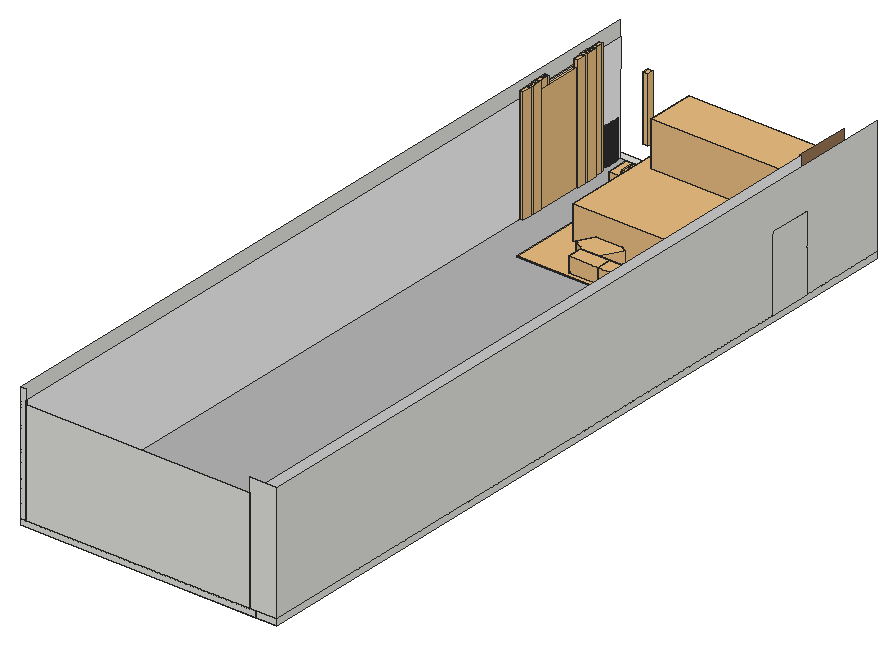
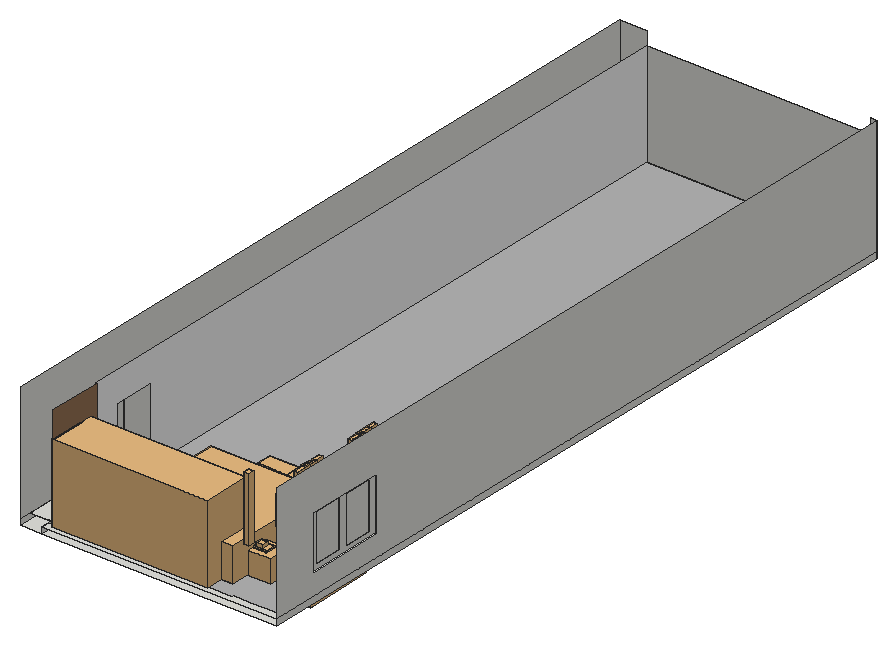
# SketchUp Ruby script. Lengths in inches.
U = 1.inch
M = Sketchup.active_model
def pt(a) = Geom::Point3d.new(a.map { |v| v * U })
def face(e, loops, mat)
  f = e.add_face(loops[0].map { |a| pt(a) })
  loops[1..].each { |l| e.add_face(l.map { |a| pt(a) }).erase! }
  f.material = f.back_material = mat if mat
  f
end
# faces: each face lists its corners as indices into pts; further lists are holes
def faces(e, pts, list, mat = nil) = list.each { |f| face(e, (f[0].is_a?(Array) ? f : [f]).map { |l| l.map { |i| pts[i] } }, mat) }
# xy, xz, yz: faces in a plane at the given z, y or x. An outline is a flat list of corners, or four numbers for a rectangle; further outlines are holes
def ring(l) = l.size == 4 ? [[l[0], l[1]], [l[2], l[1]], [l[2], l[3]], [l[0], l[3]]] : l.each_slice(2).to_a
def flat(e, list, mat, &to3) = list.each { |f| face(e, (f[0].is_a?(Array) ? f : [f]).map { |l| ring(l).map { |u, v| to3.(u, v) } }, mat) }
def xy(e, z, list, mat = nil) = flat(e, list, mat) { |x, y| [x, y, z] }
def xz(e, y, list, mat = nil) = flat(e, list, mat) { |x, z| [x, y, z] }
def yz(e, x, list, mat = nil) = flat(e, list, mat) { |y, z| [x, y, z] }
def lines(e, pts, list) = list.each { |a, b| e.add_line(pt(pts[a]), pt(pts[b])) }
# prism: a flat outline (further loops are holes) pulled along v
def prism(e, loops, v, mat = nil)
  f = face(e, loops, mat); d = Geom::Vector3d.new(v.map { |x| x * U })
  f.pushpull(f.normal.samedirection?(d) ? d.length : -d.length)
end
def box(e, o, s, mat = nil) = prism(e, [[o, [o[0] + s[0], o[1], o[2]], [o[0] + s[0], o[1] + s[1], o[2]], [o[0], o[1] + s[1], o[2]]]], [0, 0, s[2]], mat)
def at(x, y, z, deg = 0) = Geom::Transformation.translation(pt([x, y, z])) * Geom::Transformation.rotation(ORIGIN, Z_AXIS, deg.degrees)
def axes(o, x, y, z) = Geom::Transformation.new([*x, 0, *y, 0, *z, 0, *pt(o).to_a, 1])
def part(name) = M.definitions.add(name)
# library, detail: a bought-in or finely detailed component or shape, given as its bounding box
def library(name, o, s) = part(name).tap { |d| box(d.entities, o, s) }
def detail(e, o, s) = box(e.add_group.entities, o, s)
def put(e, d, t, mat = nil) = e.add_instance(d, t).tap { |i| i.material = mat if mat }
def group(e, t, mat = nil) = e.add_group.tap { |g| g.transformation = t; g.material = mat if mat }.entities
root = M.entities
M.materials.add("Carpet_Loop_Low").color = [201, 172, 127]
M.materials["Carpet_Loop_Low"].alpha = 0.3
M.materials.add("ChenZc-200606-DCZ97").color = [45, 44, 41]
M.materials.add("Generic\#1").color = [181, 181, 181]
M.materials.add("Material~1").color = [0, 0, 0]
M.materials.add("[0105_Navy]").color = [62, 69, 128]
M.materials.add("[0129_WhiteSmoke]").color = [245, 245, 245]
M.materials.add("[0130_Gainsboro]").color = [220, 220, 220]
M.materials.add("[0137_Black]").color = [0, 0, 0]
M.materials.add("[Color A01]").color = [255, 204, 204]
M.materials.add("[Color M05]").color = [114, 114, 114]
M.materials.add("[Color_001]").color = [196, 196, 196]
M.materials["[Color_001]"].alpha = 0.97
M.materials.add("[Polished Concrete New]").color = [200, 200, 203]
M.materials.add("[Wood Floor]").color = [153, 117, 86]
c1 = library("Component\#38",[0,0,0],[64.75,15.22,2.9375])
c2 = library("Upholstered bench",[-0.625,0,-2.8],[33.5,17.01,17.3])
c3 = library("Group73\#2",[-242.83,-1394.05,-548.89],[487.85,171.35,750.9])
c4 = library("Group74\#2",[-371.64,-166.22,-28.91],[497.13,332.44,58.97])
c5 = library("Group80",[524.42,-273.19,102.05],[657.62,664.02,265.78])
c6 = part("Fluted wall panel")
p = [[5.51,1.25,0],[5.9,0.93,0],[4.95,2.09,0],[5.1875,1.64,0],[6.35,0.69,0],[6.83,0.55,0],
  [7.33,0.5,0],[7.84,0.55,0],[8.32,0.69,0],[8.77,0.93,0],[9.16,1.25,0],[9.48,1.64,0],
  [9.72,2.09,0],[10,2.61,0],[10.375,3.0625,0],[10.83,3.4375,0],[17.64,0.16,0],[18.27,0.1,0],
  [11.35,3.71,0],[11.92,3.89,0],[12.51,3.94,0],[13.09,3.89,0],[20.56,1.04,0],[20.96,1.53,0],
  [13.66,3.71,0],[14.18,3.4375,0],[14.64,3.0625,0],[15.01,2.61,0],[15.29,2.09,0],[15.59,1.53,0],
  [15.99,1.04,0],[16.48,0.64,0],[17.04,0.34,0],[18.9,0.16,0],[19.51,0.34,0],[20.07,0.64,0],
  [21.26,2.09,0],[21.56,2.64,0],[21.96,3.13,0],[22.45,3.53,0],[23,3.83,0],[23.61,4.01,0],
  [24.24,4.08,0],[24.25,3.98,0]]
lines(c6.entities,p,[[0,1],[2,3],[3,0],[1,4],[4,5],[5,6],[6,7],[7,8],[8,9],[9,10],[10,11],[11,12],
  [12,13],[13,14],[14,15],[16,17],[15,18],[18,19],[19,20],[20,21],[22,23],[21,24],[24,25],[25,26],
  [26,27],[27,28],[28,29],[29,30],[30,31],[31,32],[32,16],[17,33],[33,34],[34,35],[35,22],[23,36],
  [36,37],[37,38],[38,39],[39,40],[40,41],[41,42],[42,43]])
detail(c6.entities,[0.85,0,0],[23.4,3.98,78.74])
c7 = library("组\#2",[0,0,0],[117.15,80.91,0.37])
c8 = part("Window (3)")
xy(c8.entities,31.72,[[-0.78,88.6,2.72,128.1]])
xy(c8.entities,34.95,[[-0.78,91.53,0.84,106.59],[0.84,91.53,1.05,97.58],[1.05,91.53,1.42,106.59],[1.42,91.53,2.72,106.59],[0.84,97.58,1.05,98.18],
  [0.84,98.18,1.05,106.59]])
xy(c8.entities,35.27,[[-0.78,110.09,0.97,125.14],[1.05,110.09,2.72,125.14]])
xy(c8.entities,58.35,[[2.72,108.74,3.8,109.74]])
xy(c8.entities,77.8125,[[-0.78,110.09,2.72,125.14],[0.97,110.09,1.05,125.14]])
xy(c8.entities,77.93,[[-0.78,91.53,0.84,106.59],[1.05,91.53,1.42,106.59],[1.42,91.53,2.72,106.59]])
xy(c8.entities,80.72,[[-0.78,88.6,2.72,128.1]])
xz(c8.entities,88.6,[[-0.78,31.72,2.72,80.72]])
xz(c8.entities,91.53,[[-0.78,34.95,0.84,77.93],[1.05,34.95,1.42,77.93],[1.42,34.95,2.72,77.93]])
xz(c8.entities,106.59,[[-0.78,34.95,0.84,77.93],[0.84,34.95,1.05,77.93],[0.84,34.95,2.72,77.93]])
xz(c8.entities,108.74,[[3.8,54.35,4.22,54.6,4.22,59.47,2.72,59.97,2.72,58.35,3.8,58.35]])
xz(c8.entities,109.74,[[3.8,54.35,3.8,58.35,2.72,58.35,2.72,59.97,4.22,59.47,4.22,54.6]])
xz(c8.entities,110.09,[[-0.78,35.27,0.97,77.8125],[1.05,35.27,2.72,77.8125]])
xz(c8.entities,125.14,[[-0.78,35.27,0.97,77.8125],[0.97,35.27,1.05,80.72],[1.05,35.27,2.72,77.8125]])
xz(c8.entities,128.1,[[-0.78,31.72,2.72,80.72]])
yz(c8.entities,-0.78,[[[88.6,31.72,128.1,80.72],[91.53,34.95,106.59,77.93],[110.09,35.27,125.14,77.8125]]])
yz(c8.entities,0.84,[[91.53,34.95,106.59,77.93]])
yz(c8.entities,0.97,[[110.09,35.27,125.14,77.8125]])
yz(c8.entities,1.05,[[91.53,34.95,106.59,77.93],[110.09,35.27,125.14,77.8125]])
yz(c8.entities,1.42,[[91.53,34.95,106.59,77.93]])
yz(c8.entities,2.72,[[[88.6,31.72,108.35,80.72],[91.53,34.95,106.59,77.93]],[[108.35,31.72,128.1,80.72],[110.09,35.27,125.14,77.8125],[108.74,58.35,109.74,59.97]]])
yz(c8.entities,3.8,[[108.74,54.35,109.74,58.35]])
yz(c8.entities,4.22,[[108.74,54.6,109.74,59.47]])
p = [[4.22,108.74,54.6],[3.8,108.74,54.35],[3.8,109.74,54.35],[4.22,109.74,54.6],[2.72,109.74,59.97],[2.72,108.74,59.97],
  [4.22,108.74,59.47],[4.22,109.74,59.47],[-0.78,86.4,89.94],[-0.78,86.44,89.94],[15.22,130.69,89.94],[15.22,130.65,89.94],
  [-0.78,86.44,28.19],[-0.78,86.4,28.19],[7.72,130.69,89.94],[7.72,130.65,89.94]]
faces(c8.entities,p,[[0,1,2,3],[4,5,6,7]])
lines(c8.entities,p,[[8,9],[10,11],[12,13],[14,15]])
c9 = library("3DGeom~1_Defintion\#7",[122.66,-414.5625,-71.91],[799.29,1000,104.01])
c10 = part("Group9\#3")
put(c10.entities,c9,axes([11.875,801.95,874.35],[0,-1.454,0],[0,0,2.10433],[-1.32595,0,0]),"Material~1")
c11 = part("Group8\#3")
put(c11.entities,c10,at(0,0,0))
c12 = library("@05-床_01.第一季_组\#8",[0,0,0],[98.46,95.44,37.59])
c13 = library("Group68\#1",[-167.83,-430.625,-1475.1875],[237.96,44,300])
c14 = library("组\#1",[0,0,0],[23.67,16.93,17.45])
c15 = library("Group69\#1",[-161.55,-462.88,-1311.24],[231.68,35.74,267.26])
c16 = library("Group67\#1",[-2553.52,-1371.9,-99.68],[199.61,250.46,199.36])
c17 = library("Group\#220",[-0.5,-0.5,0],[6.83,6.83,5.83])
c18 = library("Group2724",[98.25,-54.48,0.14],[27.375,24.37,69.91])
c19 = library("Group2726",[111.21,-59.05,-0.04],[18.46,18.45,1.77])
c20 = library("Group\#225",[-0.5,-0.5,0],[159.17,49.0625,79.75])
c21 = library("Pendant light",[0,0,-11.42],[5.04,6.3,65.75])
c22 = part("Fluted wall panel \#1")
p = [[3.89,0,0],[2.82,0.1,0],[2.82,0.1,33.65],[3.89,0,33.65],[4.12,0.01,0],[4.12,0.01,33.65],
  [4.34,0.02,0],[4.34,0.02,33.65],[4.97,0.04,0],[4.97,0.04,33.65],[6,0.22,0],[6,0.22,33.65],
  [12.16,0,0],[11.09,0.1,0],[11.09,0.1,33.65],[12.16,0,33.65],[12.38,0.01,0],[12.38,0.01,33.65],
  [12.61,0.02,0],[12.61,0.02,33.65],[13.24,0.04,0],[13.24,0.04,33.65],[14.27,0.22,0],[14.27,0.22,33.65],
  [1.85,0.33,0],[1.85,0.33,33.65],[10.11,0.33,0],[10.11,0.33,33.65],[6.89,0.53,0],[6.89,0.53,33.65],
  [15.16,0.53,0],[15.16,0.53,33.65],[1.02,0.6875,0],[1.02,0.6875,33.65],[9.29,0.6875,0],[9.29,0.6875,33.65],
  [7.6,0.94,0],[7.6,0.94,33.65],[15.87,0.94,0],[15.87,0.94,33.65],[0.41,1.14,0],[0.41,1.14,33.65],
  [8.68,1.14,0],[8.68,1.14,33.65],[8.07,1.43,0],[8.07,1.43,33.65],[16.34,1.43,0],[16.34,1.43,33.65],
  [0.05,1.65,0],[0.05,1.65,33.65],[8.32,1.65,0],[8.32,1.65,33.65],[8.27,1.96,0],[8.27,1.96,33.65],
  [16.54,1.96,0],[16.54,1.96,33.65],[0,1.96,33.65],[0,1.96,0],[16.55,2.08,33.65],[16.55,2.08,33.35],
  [16.55,2.08,18.875],[16.55,2.08,7.8],[16.55,2.08,0]]
faces(c22.entities,p,[[0,1,2,3],[4,0,3,5],[6,4,5,7],[8,6,7,9],[10,8,9,11],[12,13,14,15],[16,12,15,17],[18,16,17,19],
  [20,18,19,21],[22,20,21,23],[1,24,25,2],[13,26,27,14],[28,10,11,29],[30,22,23,31],[24,32,33,25],[26,34,35,27],
  [36,28,29,37],[38,30,31,39],[32,40,41,33],[34,42,43,35],[44,36,37,45],[46,38,39,47],[40,48,49,41],[42,50,51,43],
  [52,44,45,53],[54,46,47,55],[56,49,48,57],[53,51,50,52],[55,58,59,60,61,62,54]],"[0105_Navy]")
c23 = part("Fluted wall panel \#2")
p = [[3.89,0,0],[2.82,0.1,0],[2.82,0.1,33.65],[3.89,0,33.65],[4.12,0.01,0],[4.12,0.01,33.65],
  [4.34,0.02,0],[4.34,0.02,33.65],[4.97,0.04,0],[4.97,0.04,33.65],[6,0.22,0],[6,0.22,33.65],
  [12.16,0,0],[11.09,0.1,0],[11.09,0.1,33.65],[12.16,0,33.65],[12.38,0.01,0],[12.38,0.01,33.65],
  [12.61,0.02,0],[12.61,0.02,33.65],[13.24,0.04,0],[13.24,0.04,33.65],[14.27,0.22,0],[14.27,0.22,33.65],
  [1.85,0.33,0],[1.85,0.33,33.65],[10.11,0.33,0],[10.11,0.33,33.65],[6.89,0.53,0],[6.89,0.53,33.65],
  [15.16,0.53,0],[15.16,0.53,33.65],[1.02,0.6875,0],[1.02,0.6875,33.65],[9.29,0.6875,0],[9.29,0.6875,33.65],
  [7.6,0.94,0],[7.6,0.94,33.65],[15.87,0.94,0],[15.87,0.94,33.65],[0.41,1.14,0],[0.41,1.14,33.65],
  [8.68,1.14,0],[8.68,1.14,33.65],[8.07,1.43,0],[8.07,1.43,33.65],[16.34,1.43,0],[16.34,1.43,33.65],
  [0.05,1.65,0],[0.05,1.65,33.65],[8.32,1.65,0],[8.32,1.65,33.65],[8.27,1.96,0],[8.27,1.96,33.65],
  [16.54,1.96,0],[16.54,1.96,33.65],[0,1.96,33.65],[0,1.96,0],[16.55,2.08,33.65],[16.55,2.08,33.35],
  [16.55,2.08,18.875],[16.55,2.08,7.8],[16.55,2.08,0]]
faces(c23.entities,p,[[0,1,2,3],[4,0,3,5],[6,4,5,7],[8,6,7,9],[10,8,9,11],[12,13,14,15],[16,12,15,17],[18,16,17,19],
  [20,18,19,21],[22,20,21,23],[1,24,25,2],[13,26,27,14],[28,10,11,29],[30,22,23,31],[24,32,33,25],[26,34,35,27],
  [36,28,29,37],[38,30,31,39],[32,40,41,33],[34,42,43,35],[44,36,37,45],[46,38,39,47],[40,48,49,41],[42,50,51,43],
  [52,44,45,53],[54,46,47,55],[56,49,48,57],[53,51,50,52],[55,58,59,60,61,62,54]],"[0105_Navy]")
xy(root,40.281,[[0,0,240,763.0625],[240,0,261.625,763.0625]])
xy(root,46.281,[[0,0,6,0,6,755.5,19.81,755.5,19.81,755.8125,20.995,755.8125,20.995,755.5,27.258,755.5,27.258,755.8125,28.492,755.8125,28.492,755.5,50.612,755.5,50.612,756.6875,75.457,756.6875,75.457,755.5,180.702,755.5,180.702,756.3125,181.219,756.3125,181.219,755.5,182.702,755.5,182.702,756.3125,183.219,756.3125,183.219,755.5,184.702,755.5,184.702,756.3125,185.219,756.3125,185.219,755.5,186.702,755.5,186.702,756.3125,187.219,756.3125,187.219,755.5,188.702,755.5,188.702,756.3125,189.219,756.3125,189.219,755.5,190.702,755.5,190.702,756.3125,191.219,756.3125,191.219,755.5,192.702,755.5,192.702,756.3125,193.219,756.3125,193.219,755.5,194.702,755.5,194.702,756.3125,195.219,756.3125,195.219,755.5,196.702,755.5,196.702,756.3125,197.219,756.3125,197.219,755.5,198.702,755.5,198.702,756.3125,199.219,756.3125,199.219,755.5,200.702,755.5,200.702,756.3125,201.219,756.3125,201.219,755.5,202.702,755.5,202.702,756.3125,203.219,756.3125,203.219,755.5,204.702,755.5,204.702,756.3125,205.219,756.3125,205.219,755.5,206.702,755.5,206.702,756.3125,207.219,756.3125,207.219,755.5,208.702,755.5,208.702,755.8125,209.219,755.8125,209.219,755.5,210.702,755.5,210.702,755.8125,211.219,755.8125,211.219,755.5,232.4375,755.5,232.4375,754.006,240,754.006,240,763.0625,0,763.0625],[234,0,240,631.303],[240,0,261.625,631.303],[240,631.303,261.625,674.116],[233.0625,674.116,240,674.116,240,751.105,234,751.105,234,709.314,233.0625,709.314],
  [240,674.116,261.625,751.105],[232.4375,709.314,234,751.105],[240,751.105,241.336,751.105,240.269,751.205,240,751.269],[241.336,751.105,242.418,751.147,243.115,751.269,240,751.269,240.269,751.205],[241.336,751.105,261.625,751.105,261.625,751.269,243.115,751.269,242.418,751.147]])
xy(root,46.281,[[6,0,234,0,234,631.303,240,631.303,240,674.116,233.0625,674.116,233.0625,709.314,232.4375,709.314,232.4375,751.105,175.191,751.105,175.098,751.114,171.282,751.114,171.282,753.181,171.265,753.406,171.282,753.498,171.282,754.006,232.4375,754.006,232.4375,755.5,211.219,755.5,211.219,755.8125,210.702,755.8125,210.702,755.5,209.219,755.5,209.219,755.8125,208.702,755.8125,208.702,755.5,207.219,755.5,207.219,756.3125,206.702,756.3125,206.702,755.5,205.219,755.5,205.219,756.3125,204.702,756.3125,204.702,755.5,203.219,755.5,203.219,756.3125,202.702,756.3125,202.702,755.5,201.219,755.5,201.219,756.3125,200.702,756.3125,200.702,755.5,199.219,755.5,199.219,756.3125,198.702,756.3125,198.702,755.5,197.219,755.5,197.219,756.3125,196.702,756.3125,196.702,755.5,195.219,755.5,195.219,756.3125,194.702,756.3125,194.702,755.5,193.219,755.5,193.219,756.3125,192.702,756.3125,192.702,755.5,191.219,755.5,191.219,756.3125,190.702,756.3125,190.702,755.5,189.219,755.5,189.219,756.3125,188.702,756.3125,188.702,755.5,187.219,755.5,187.219,756.3125,186.702,756.3125,186.702,755.5,185.219,755.5,185.219,756.3125,184.702,756.3125,184.702,755.5,183.219,755.5,183.219,756.3125,182.702,756.3125,182.702,755.5,181.219,755.5,181.219,756.3125,180.702,756.3125,180.702,755.5,75.457,755.5,75.457,756.6875,50.612,756.6875,50.612,755.5,28.492,755.5,28.492,755.8125,27.258,755.8125,27.258,755.5,20.995,755.5,20.995,755.8125,19.81,755.8125,19.81,755.5,6,755.5]],"Generic\#1")
xy(root,46.281,[[175.191,751.105,175.416,751.114,175.098,751.114],[199.995,751.105,208.263,751.105,207.197,751.205,206.218,751.439,205.394,751.793,204.781,752.24,204.42,752.752,204.372,753.068,204.172,752.535,203.703,752.045,202.997,751.633,202.101,751.327,201.077,751.147,200.446,751.122,200.22,751.114],[208.263,751.105,216.531,751.105,215.465,751.205,214.486,751.439,213.662,751.793,213.049,752.24,212.688,752.752,212.64,753.068,212.44,752.535,211.971,752.045,211.265,751.633,210.369,751.327,209.345,751.147,208.714,751.122,208.489,751.114],[224.8,751.105,225.025,751.114,225.25,751.122,225.882,751.147,226.905,751.327,227.801,751.633,228.507,752.045,228.976,752.535,229.176,753.068,229.225,752.752,229.585,752.24,230.198,751.793,231.022,751.439,232.001,751.205,232.4375,751.164,232.4375,751.105],[232.4375,751.105,232.4375,751.164,233.068,751.105],
  [233.068,751.105,234,751.105,234,751.141,233.518,751.122,233.293,751.114]],"[Color A01]")
xy(root,50.281,[[233.0625,674.116,234,700.967],[234,674.116,261.625,675.053],[233.0625,700.967,233.625,709.314]],"[Color M05]")
xy(root,67.912,[[0,635.766,6,717.204]])
xz(root,0,[[0,40.281,240,46.281],[240,40.281,261.625,46.281],[0,46.281,6,166.281],[6,46.281,234,46.281,234,152.123,6.399,152.123,6.399,155.498,6,155.498],[234,46.281,261.625,166.281]])
xz(root,631.303,[[234,46.281,261.625,122.281]])
xz(root,635.766,[[0,67.912,6,123.475]])
xz(root,674.116,[[233.0625,46.281,261.625,50.281]],"[Color M05]")
xz(root,675.053,[[234,50.281,261.625,122.281]])
xz(root,700.967,[[233.625,50.281,234,152.123]])
xz(root,709.314,[[233.0625,46.281,234,50.281],[233.625,50.281,234,111.518]])
xz(root,709.314,[[232.4375,46.281,233.0625,46.281,233.0625,50.281,233.031,50.281,233.031,111.518,232.4375,111.518]],"[Polished Concrete New]")
xz(root,717.204,[[0,67.912,6,123.475]])
yz(root,0,[[0,40.281,763.0625,46.281],[[0,46.281,763.0625,166.281],[635.766,67.912,717.204,123.475]]])
yz(root,6,[[[0,46.281,755.5,46.281,755.5,126.503,756.6875,126.503,756.6875,155.498,0,155.498],[635.766,67.912,717.204,123.475]]],"[0129_WhiteSmoke]")
yz(root,232.4375,[[709.314,46.281,709.314,111.518,709.438,113.412,709.808,115.274,710.418,117.071,711.258,118.774,712.312,120.352,713.564,121.779,714.991,123.031,716.569,124.085,718.272,124.925,720.069,125.535,721.931,125.905,723.825,126.029,755.5,126.029,755.5,46.281]],"[0130_Gainsboro]")
yz(root,233.0625,[[674.116,46.281,709.314,50.281]],"[Color M05]")
yz(root,233.625,[[700.967,50.281,700.967,152.123,756.6875,152.123,756.6875,126.029,723.825,126.029,721.931,125.905,720.069,125.535,718.272,124.925,716.569,124.085,714.991,123.031,713.564,121.779,712.312,120.352,711.258,118.774,710.418,117.071,709.808,115.274,709.438,113.412,709.314,111.518,709.314,50.281]],"[Wood Floor]")
yz(root,234,[[709.314,46.281,709.314,111.518,709.438,113.412,709.808,115.274,710.418,117.071,711.258,118.774,712.312,120.352,713.564,121.779,714.991,123.031,716.569,124.085,718.272,124.925,720.069,125.535,721.931,125.905,723.825,126.029,757.0625,126.029,757.0625,46.281]])
yz(root,234,[[0,46.281,0,152.123,700.967,152.123,700.967,50.281,675.053,50.281,675.053,122.281,631.303,122.281,631.303,46.281]],"[0129_WhiteSmoke]")
yz(root,240,[[0,40.281,763.0625,46.281]])
yz(root,261.625,[[0,40.281,763.0625,46.281],[0,46.281,631.303,46.281,631.303,122.281,675.053,122.281,675.053,50.281,674.116,50.281,674.116,46.281,763.0625,46.281,763.0625,166.281,0,166.281],[631.303,46.281,674.116,122.281],[674.116,50.281,675.053,122.281]])
p = [[175.098,751.114,46.281],[174.124,751.205,46.281],[174.124,751.205,84.304],[175.191,751.105,84.304],[175.191,751.105,46.281],[175.416,751.114,46.281],
  [175.416,751.114,84.304],[175.641,751.122,46.281],[175.641,751.122,84.304],[176.273,751.147,46.281],[176.273,751.147,84.304],[177.297,751.327,46.281],
  [177.297,751.327,84.304],[183.459,751.105,46.281],[182.392,751.205,46.281],[182.392,751.205,84.304],[183.459,751.105,84.304],[183.684,751.114,46.281],
  [183.684,751.114,84.304],[183.909,751.122,46.281],[183.909,751.122,84.304],[184.541,751.147,46.281],[184.541,751.147,84.304],[185.565,751.327,46.281],
  [185.565,751.327,84.304],[191.727,751.105,46.281],[190.66,751.205,46.281],[190.66,751.205,84.304],[191.727,751.105,84.304],[191.952,751.114,46.281],
  [191.952,751.114,84.304],[192.178,751.122,46.281],[192.178,751.122,84.304],[192.809,751.147,46.281],[192.809,751.147,84.304],[193.833,751.327,46.281],
  [193.833,751.327,84.304],[199.995,751.105,46.281],[198.928,751.205,46.281],[198.928,751.205,84.304],[199.995,751.105,84.304],[200.22,751.114,46.281],
  [200.22,751.114,84.304],[200.446,751.122,46.281],[200.446,751.122,84.304],[201.077,751.147,46.281],[201.077,751.147,84.304],[202.101,751.327,46.281],
  [202.101,751.327,84.304],[208.263,751.105,46.281],[207.197,751.205,46.281],[207.197,751.205,84.304],[208.263,751.105,84.304],[208.489,751.114,46.281],
  [208.489,751.114,84.304],[208.714,751.122,46.281],[208.714,751.122,84.304],[209.345,751.147,46.281],[209.345,751.147,84.304],[210.369,751.327,46.281],
  [210.369,751.327,84.304],[216.531,751.105,46.281],[215.465,751.205,46.281],[215.465,751.205,84.304],[216.531,751.105,84.304],[216.757,751.114,46.281],
  [216.757,751.114,84.304],[216.982,751.122,46.281],[216.982,751.122,84.304],[217.614,751.147,46.281],[217.614,751.147,84.304],[218.637,751.327,46.281],
  [218.637,751.327,84.304],[224.8,751.105,46.281],[223.733,751.205,46.281],[223.733,751.205,84.304],[224.8,751.105,84.304],[225.025,751.114,46.281],
  [225.025,751.114,84.304],[225.25,751.122,46.281],[225.25,751.122,84.304],[225.882,751.147,46.281],[225.882,751.147,84.304],[226.905,751.327,46.281],
  [226.905,751.327,84.304],[232.4375,751.164,46.281],[232.001,751.205,46.281],[232.001,751.205,84.304],[233.068,751.105,84.304],[233.068,751.105,46.281],
  [233.293,751.114,46.281],[233.293,751.114,84.304],[233.518,751.122,46.281],[233.518,751.122,84.304],[234,751.141,46.281],[234.15,751.147,84.304],
  [234.15,751.147,46.281],[235.174,751.327,46.281],[235.174,751.327,84.304],[173.145,751.439,46.281],[173.145,751.439,84.304],[181.413,751.439,46.281],
  [181.413,751.439,84.304],[189.682,751.439,46.281],[189.682,751.439,84.304],[197.95,751.439,46.281],[197.95,751.439,84.304],[206.218,751.439,46.281],
  [206.218,751.439,84.304],[214.486,751.439,46.281],[214.486,751.439,84.304],[222.754,751.439,46.281],[222.754,751.439,84.304],[231.022,751.439,46.281],
  [231.022,751.439,84.304],[178.192,751.633,46.281],[178.192,751.633,84.304],[186.46,751.633,46.281],[186.46,751.633,84.304],[194.728,751.633,46.281],
  [194.728,751.633,84.304],[202.997,751.633,46.281],[202.997,751.633,84.304],[211.265,751.633,46.281],[211.265,751.633,84.304],[219.533,751.633,46.281],
  [219.533,751.633,84.304],[227.801,751.633,46.281],[227.801,751.633,84.304],[236.069,751.633,46.281],[236.069,751.633,84.304],[172.321,751.793,46.281],
  [172.321,751.793,84.304],[180.589,751.793,46.281],[180.589,751.793,84.304],[188.858,751.793,46.281],[188.858,751.793,84.304],[197.126,751.793,46.281],
  [197.126,751.793,84.304],[205.394,751.793,46.281],[205.394,751.793,84.304],[213.662,751.793,46.281],[213.662,751.793,84.304],[221.93,751.793,46.281],
  [221.93,751.793,84.304],[230.198,751.793,46.281],[230.198,751.793,84.304],[238.466,751.793,79.929],[239.29,751.439,79.929],[240.269,751.205,79.929],
  [241.336,751.105,79.929],[9.674,709.072,46.281],[9.674,709.072,163.21],[9.948,716.257,163.21],[9.948,716.257,46.281],[243.115,751.269,46.281],
  [243.442,751.327,46.281],[145.053,623.394,47.325],[93.615,623.394,47.325]]
faces(root,p,[[0,1,2,3,4],[5,4,3,6],[7,5,6,8],[9,7,8,10],[11,9,10,12],[13,14,15,16],[17,13,16,18],[19,17,18,20],
  [21,19,20,22],[23,21,22,24],[25,26,27,28],[29,25,28,30],[31,29,30,32],[33,31,32,34],[35,33,34,36],[37,38,39,40],
  [41,37,40,42],[43,41,42,44],[45,43,44,46],[47,45,46,48],[49,50,51,52],[53,49,52,54],[55,53,54,56],[57,55,56,58],
  [59,57,58,60],[61,62,63,64],[65,61,64,66],[67,65,66,68],[69,67,68,70],[71,69,70,72],[73,74,75,76],[77,73,76,78],
  [79,77,78,80],[81,79,80,82],[83,81,82,84],[85,86,87,88,89],[90,89,88,91],[92,90,91,93],[94,92,93,95,96],[97,96,95,98],
  [1,99,100,2],[14,101,102,15],[26,103,104,27],[38,105,106,39],[50,107,108,51],[62,109,110,63],[74,111,112,75],[86,113,114,87],
  [115,11,12,116],[117,23,24,118],[119,35,36,120],[121,47,48,122],[123,59,60,124],[125,71,72,126],[127,83,84,128],[129,97,98,130],
  [99,131,132,100],[101,133,134,102],[103,135,136,104],[105,137,138,106],[107,139,140,108],[109,141,142,110],[111,143,144,112],[113,145,146,114]],"[0105_Navy]")
lines(root,p,[[147,148],[148,149],[149,150],[151,152],[153,154],[155,156],[157,158]])
detail(root,[169.55,716.59,80.13],[3.91,3.91,2.58])
put(root,c1,axes([93.5625,583.08,47.77],[0.89,0,0],[0,0.89,0],[0,0,0.89]),"[0137_Black]")
put(root,c2,axes([93.12,582.33,49.82],[0.89,0,0],[0,0.89,0],[0,0,0.89]))
put(root,c2,axes([151.63,582.33,49.82],[-0.89,0,0],[0,0.89,0],[0,0,0.89]))
put(root,c3,axes([164.87,611.52,108.86],[-0.01858,0.03985,0],[0,0,0.04397],[0.03985,0.01858,0]))
put(root,c4,axes([122.92,609.72,48.17],[-0.04071,0.01091,-0.00301],[0.01093,0.04078,0],[-0.00235,0.00063,0.05214]))
put(root,c5,axes([132.98,598.47,42.79],[-0.03933,0.02271,0],[-0.02271,-0.03933,0],[0,0,0.04541]))
put(root,c6,axes([6,627.66,46.28],[0,0.3942,0],[1,0,0],[0,0,1.485]),"Carpet_Loop_Low")
put(root,c7,axes([43.19,578.47,47.07],[1.32063,0,0],[0,1.44926,0],[0,0,-2.14862]))
put(root,c6,axes([5.91,635.86,46.28],[0,0.3942,0],[1,0,0],[0,0,1.485]),"Carpet_Loop_Low")
put(root,c6,axes([6,640.91,46.28],[0,0.3942,0],[1,0,0],[0,0,1.485]),"Carpet_Loop_Low")
put(root,c6,axes([4.8125,645.01,46.28],[0,0.69281,0],[1,0,0],[0,0,1.485]),"Carpet_Loop_Low")
g1 = group(root,at(155.18,654.4,46.89))
xy(g1,0,[[-1.56,-1.625,1.56,1.625]],"ChenZc-200606-DCZ97")
xy(g1,1.53,[[-1.77,-1.85,1.77,1.85]],"ChenZc-200606-DCZ97")
p = [[1.77,-1.85,1.53],[1.56,-1.625,0],[-1.56,-1.625,0],[-1.77,-1.85,1.53],[-1.56,1.625,0],[-1.77,1.85,1.53],
  [1.77,1.85,1.53],[1.56,1.625,0]]
faces(g1,p,[[0,1,2,3],[3,2,4,5],[6,7,1,0],[5,4,7,6]],"ChenZc-200606-DCZ97")
put(root,c6,axes([4.87,649.6875,46.28],[0,0.3942,0],[1,0,0],[0,0,1.485]),"Carpet_Loop_Low")
put(root,c8,axes([3.28,453.13,32.08],[1,0,0],[0,2.06187,0],[0,0,1.1322]))
put(root,c11,axes([8.28,677.1,34.27],[-0.03519,0,0],[0,0.06098,0],[0,0,0.05732]),"[Color_001]")
put(root,c12,axes([62.48,624.92,47.11],[1.17056,0,0],[0,1.21594,0],[0,0,0.90756]))
put(root,c6,axes([7.26,695.59,46.28],[0,0.3942,0],[1,0,0],[0,0,1.485]),"Carpet_Loop_Low")
put(root,c6,axes([6.125,704.37,46.28],[0,0.3942,0],[1,0,0],[0,0,1.485]),"Carpet_Loop_Low")
put(root,c13,axes([-16.27,708.27,85.24],[0,-0.04859,0],[0,0,0.03946],[-0.05499,0,0]))
put(root,c14,axes([39.58,699.41,46.28],[1.34118,0,0],[0,1.34118,0],[0,0,1.34118]))
put(root,c15,axes([-16.22,709.05,86.67],[0,-0.04439,0],[0,0,0.03598],[-0.06186,0,0]))
put(root,c16,axes([-22.4,712.18,89.65],[-0.03202,0,0],[0,0,0.01336],[0,-0.03216,0]))
put(root,c6,axes([7.26,708.84,46.28],[0,0.3942,0],[1,0,0],[0,0,1.485]),"Carpet_Loop_Low")
put(root,c17,axes([173.26,716.85,78.39],[0,0.60715,0],[-0.60715,0,0],[0,0,0.60715]))
put(root,c6,axes([6.07,712.94,46.28],[0,0.69281,0],[1,0,0],[0,0,1.485]),"Carpet_Loop_Low")
put(root,c18,axes([163.54,692.87,68.25],[0,0.26,0],[-0.26,0,0],[0,0,0.26]))
put(root,c6,axes([6.125,717.62,46.28],[0,0.3942,0],[1,0,0],[0,0,1.485]),"Carpet_Loop_Low")
put(root,c19,axes([163.54,692.87,68.25],[0,0.26,0],[-0.26,0,0],[0,0,0.26]))
put(root,c14,axes([172.8,715.99,46.28],[1.34118,0,0],[0,1.34118,0],[0,0,1.34118]))
put(root,c20,at(75.46,709.3125,46.28))
put(root,c21,at(49.63,731.26,96.04))
put(root,c22,axes([230.36,752.14,46.28],[0,-1,0],[1,0,0],[0,0,1.13]),"[0105_Navy]")
put(root,c23,axes([8.08,735.76,46.28],[0,1,0],[-1,0,0],[0,0,1.13]))
